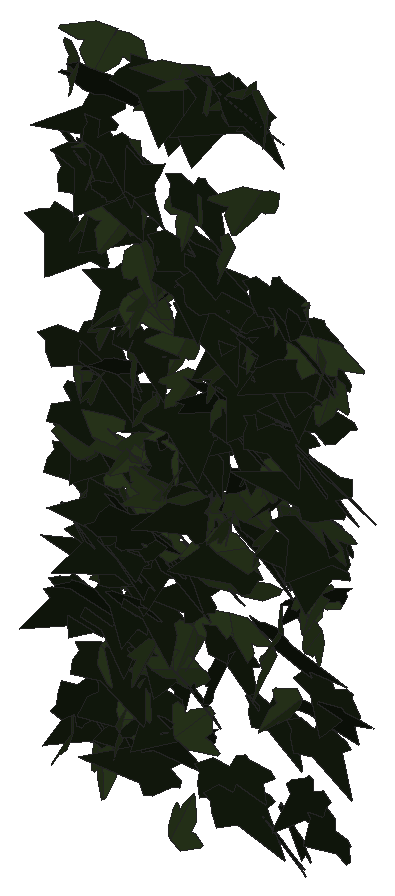
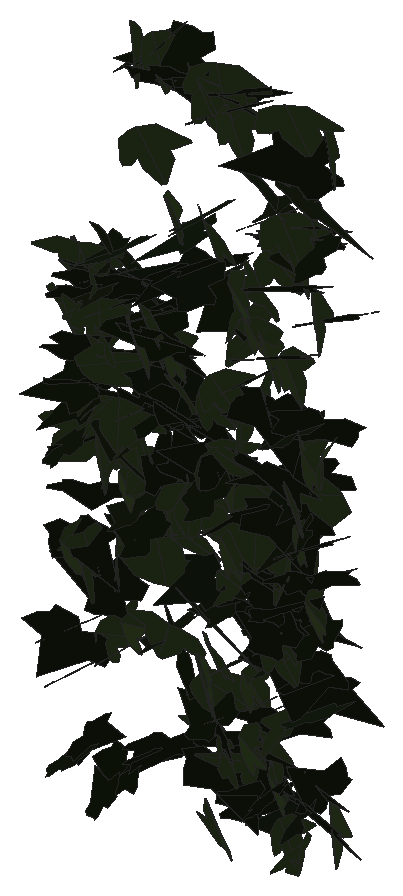
# SketchUp Ruby script. Lengths in millimetres.
U = 1.mm
M = Sketchup.active_model
def pt(a) = Geom::Point3d.new(a.map { |v| v * U })
def face(e, loops, mat)
  f = e.add_face(loops[0].map { |a| pt(a) })
  loops[1..].each { |l| e.add_face(l.map { |a| pt(a) }).erase! }
  f.material = f.back_material = mat if mat
  f
end
# faces: each face lists its corners as indices into pts; further lists are holes
def faces(e, pts, list, mat = nil) = list.each { |f| face(e, (f[0].is_a?(Array) ? f : [f]).map { |l| l.map { |i| pts[i] } }, mat) }
# xy, xz, yz: faces in a plane at the given z, y or x. An outline is a flat list of corners, or four numbers for a rectangle; further outlines are holes
def ring(l) = l.size == 4 ? [[l[0], l[1]], [l[2], l[1]], [l[2], l[3]], [l[0], l[3]]] : l.each_slice(2).to_a
def flat(e, list, mat, &to3) = list.each { |f| face(e, (f[0].is_a?(Array) ? f : [f]).map { |l| ring(l).map { |u, v| to3.(u, v) } }, mat) }
def xy(e, z, list, mat = nil) = flat(e, list, mat) { |x, y| [x, y, z] }
def xz(e, y, list, mat = nil) = flat(e, list, mat) { |x, z| [x, y, z] }
def yz(e, x, list, mat = nil) = flat(e, list, mat) { |y, z| [x, y, z] }
def lines(e, pts, list) = list.each { |a, b| e.add_line(pt(pts[a]), pt(pts[b])) }
# prism: a flat outline (further loops are holes) pulled along v
def prism(e, loops, v, mat = nil)
  f = face(e, loops, mat); d = Geom::Vector3d.new(v.map { |x| x * U })
  f.pushpull(f.normal.samedirection?(d) ? d.length : -d.length)
end
def box(e, o, s, mat = nil) = prism(e, [[o, [o[0] + s[0], o[1], o[2]], [o[0] + s[0], o[1] + s[1], o[2]], [o[0], o[1] + s[1], o[2]]]], [0, 0, s[2]], mat)
def at(x, y, z, deg = 0) = Geom::Transformation.translation(pt([x, y, z])) * Geom::Transformation.rotation(ORIGIN, Z_AXIS, deg.degrees)
def axes(o, x, y, z) = Geom::Transformation.new([*x, 0, *y, 0, *z, 0, *pt(o).to_a, 1])
def part(name) = M.definitions.add(name)
# library, detail: a bought-in or finely detailed component or shape, given as its bounding box
def library(name, o, s) = part(name).tap { |d| box(d.entities, o, s) }
def detail(e, o, s) = box(e.add_group.entities, o, s)
def put(e, d, t, mat = nil) = e.add_instance(d, t).tap { |i| i.material = mat if mat }
def group(e, t, mat = nil) = e.add_group.tap { |g| g.transformation = t; g.material = mat if mat }.entities
root = M.entities
M.materials.add("efeu1").color = [18, 25, 13]
M.materials.add("efeu2").color = [43, 57, 29]
c1 = part("ivyleaf_9")
p = [[39.1,54.8,31.7],[34.5,51.8,30.2],[-5.3,25.2,17.3],[-17.9,28.3,20.9],[-21.6,21.7,17],[-20.2,4.3,5.3],
  [-22.9,-0.3,2.5],[-17.1,-4,-0.6],[-2,-2.1,-1.2],[-0.7,-15.4,-10.1],[16.6,-22.3,-16.7],[21.1,-15.1,-12.5],
  [32.7,-10.7,-11],[46.1,-1.8,-6.6],[30.8,11.2,3.8]]
faces(c1.entities,p,[[0,1,2,3,4,5,6,7,8,9,10,11,12,13,14]],"efeu1")
c2 = part("ivyleaf_10")
p = [[0,12.8,-0.8],[-1.5,51.3,-10.9],[-4.9,51,-11.6],[-13.6,26.5,-7.3],[-13.2,15.9,-4.6],[-21.1,19.3,-7.2],
  [-29.5,16.3,-8.3],[-29.2,8.3,-6.2],[-19.7,-9.8,0.5],[-7.6,-13,4],[1,-12.2,5.8],[-0.4,51.1,-11.1],
  [-1.5,51.1,-10.9],[1,-12.4,5.9],[16.9,-12.4,3.5],[35.1,9.1,-5.1],[35,12.9,-6.1],[20.5,16.4,-4.9],
  [15.8,15,-3.8],[15.3,27.6,-7.1],[12.8,31.3,-7.8]]
faces(c2.entities,p,[[0,1,2,3,4,5,6,7,8,9,10],[11,12,0,13,14,15,16,17,18,19,20]],"efeu2")
put(root,c1,axes([3167.3,851.9,1947.2],[-1.71163,0.02943,0.11968],[-0.22866,-0.01275,-0.89967],[-0.05232,-0.90718,0.01653]))
put(root,c1,axes([3252.4,861.6,2324.2],[-0.11575,-0.94583,0.25251],[0.04501,-0.25434,-0.947],[1.8626,-0.05263,0.03857]))
put(root,c1,axes([3092.4,865,2330.9],[-0.99766,-0.72669,0.37742],[-0.1338,-0.40653,-0.8804],[1.55269,-0.50196,0.16664]))
put(root,c1,axes([3190,827.4,2438.5],[0.54104,0.53541,0.79457],[-0.52659,0.83937,-0.4666],[-1.74581,-0.08725,0.38698]))
put(root,c2,axes([3112.9,842.3,2090.9],[-0.7712,-0.10733,-1.03525],[1.96959,0.07673,-0.41303],[0.21089,-1.10908,0.07161]))
put(root,c2,axes([3164.4,858.5,2380.3],[-0.74877,-0.74862,0.505],[-0.03893,-0.54332,-0.82136],[1.71819,-0.33855,0.20146]))
put(root,c2,axes([3201.5,857.9,1829.8],[0.10736,-0.83868,0.42223],[0.20075,-0.41465,-0.83772],[1.77573,0.09758,0.06918]))
put(root,c2,axes([3199.2,856.4,2286.4],[0.21582,-0.91043,0.32112],[0.15942,-0.31283,-0.91651],[1.83043,0.13459,0.04196]))
put(root,c1,axes([3111.1,858.5,1856.1],[0.09211,0.1256,-0.88774],[-0.40662,-0.86181,-0.13358],[-1.65722,0.21844,-0.01657]))
put(root,c2,axes([3291,861.4,2056.1],[-0.08821,0.50692,-0.77285],[0.03891,-0.77307,-0.50829],[-1.75863,-0.04253,0.02752]))
put(root,c2,axes([3185.1,860,2333.8],[1.05203,-0.35932,0.77542],[1.2124,-0.44238,-0.65911],[1.08429,0.84328,-0.01536]))
put(root,c2,axes([3151.5,852.3,2249.2],[0.05261,-0.96666,0.06985],[0.05652,-0.069,-0.96666],[1.84368,0.0297,0.02764]))
put(root,c1,axes([3334.6,847.4,1688.7],[0.31329,-0.78141,-0.53609],[-0.03358,0.54149,-0.7947],[1.8032,0.14585,0.07834]))
put(root,c2,axes([3399.3,866.1,1822.8],[0.03799,-0.34084,0.87208],[0.19157,-0.86645,-0.34094],[1.77168,0.10099,0.01817]))
put(root,c2,axes([3134.6,847.1,2163.2],[0.242,-0.92573,-0.21991],[0.03708,0.22436,-0.93316],[1.8105,0.11914,0.04851]))
put(root,c2,axes([3218.8,843,2165.7],[-0.07443,-0.88003,-0.43626],[0.27149,0.42688,-0.87391],[1.84955,-0.09807,0.11072]))
put(root,c1,axes([3157.1,866.8,1871.5],[-0.13634,-0.73855,0.50918],[-0.10426,-0.50624,-0.742],[1.70409,-0.09006,-0.00466]))
put(root,c1,axes([3220.3,863.7,2574.1],[-0.82164,-0.93763,-0.01567],[0.09231,-0.0051,-1.03121],[1.78235,-0.43197,0.04618]))
put(root,c1,axes([3428.2,860.3,2277.4],[-1.7636,-0.19236,0.12728],[-0.23141,-0.04043,-0.94629],[0.37305,-0.93448,0.01474]))
put(root,c2,axes([3095.1,842,1687.4],[0.18402,-0.83212,-0.61124],[-0.10409,0.60893,-0.83762],[1.96229,0.11034,0.01289]))
put(root,c2,axes([3255,853.6,1741.5],[1.35818,-0.41325,-0.37001],[0.61897,-0.1767,0.82459],[-0.85519,-0.78419,0.00919]))
put(root,c1,axes([3169.3,841.5,1972.8],[-0.11479,-0.10418,0.94422],[1.73049,0.26763,0.08761],[-0.52352,0.9075,0.08256]))
put(root,c1,axes([3329,854.4,2597.8],[0.81855,-0.90853,-0.30046],[-0.25701,0.26849,-1.00517],[1.803,0.45074,-0.00687]))
put(root,c2,axes([3127.3,848.9,2445.7],[0.64331,-0.86532,-0.34696],[-0.13269,0.34457,-0.92727],[1.76936,0.34046,0.05661]))
put(root,c1,axes([3282.2,846.1,2369],[1.27105,-0.57956,-0.4415],[-0.26412,0.48676,-0.8489],[1.36123,0.63561,0.24754]))
put(root,c2,axes([3317.3,852.1,2387.8],[0.71463,-0.93857,-0.20251],[-0.08346,0.20046,-1.01035],[1.82548,0.37659,0.03309]))
put(root,c2,axes([3245.7,853.8,1608.1],[1.2389,-0.73981,-0.07337],[0.09338,-0.05456,0.98543],[-1.41184,-0.6528,0.00079]))
put(root,c1,axes([3320.2,870.3,1977.6],[-1.25451,-0.26857,0.61132],[-0.67706,-0.58569,-0.64089],[1.07542,-0.68203,0.30963]))
put(root,c1,axes([3277.3,854.5,2034],[-1.61102,0.36065,0.05804],[-0.10432,0.01943,-0.9201],[-0.68735,-0.84825,0.0036]))
put(root,c1,axes([3409.3,841.6,2308.2],[-0.85147,0.86442,0.32225],[-0.27728,0.28745,-0.97333],[-1.73373,-0.47051,-0.0026]))
put(root,c1,axes([3375.9,859,1813.1],[0.33026,-0.85237,-0.15761],[-0.0701,0.15334,-0.86984],[1.64824,0.17731,-0.00541]))
put(root,c2,axes([3351.6,860.1,2467.9],[-0.87179,-0.87367,0.30003],[-0.10421,-0.30863,-0.98229],[1.755,-0.45232,0.09071]))
put(root,c1,axes([3141.7,869.5,1973.7],[-0.77384,-0.07875,0.80711],[-1.07948,-0.61768,-0.346],[1.10307,-0.65971,0.22761]))
put(root,c2,axes([3182.1,853.8,2264.3],[0.35123,-0.94079,-0.16334],[-0.06352,0.15991,-0.95872],[1.81619,0.18753,-0.00194]))
put(root,c1,axes([3137.6,870.6,2431],[-1.24934,-0.74587,0.19918],[-0.11965,-0.20893,-0.98959],[1.4644,-0.6534,0.08907]))
put(root,c1,axes([3249.9,864.9,2150.7],[-0.42151,-0.95738,-0.12023],[0.06952,0.11495,-0.98262],[1.83508,-0.22426,0.00961]))
put(root,c1,axes([3154.8,858,1801.2],[-0.7348,-0.70133,-0.54457],[0.50248,0.47629,-0.80058],[1.61348,-0.46772,0.00131]))
put(root,c1,axes([3460.5,861.8,2113.7],[-1.09379,0.20172,0.72488],[-1.43095,-0.18893,-0.54353],[0.0549,-0.90556,0.27487]))
put(root,c1,axes([3284.4,860.7,2290.5],[-0.0781,-0.92797,-0.29273],[0.06005,0.29157,-0.92871],[1.85093,-0.04861,0.01778]))
put(root,c2,axes([3172.8,865.9,2209.4],[0.49749,-0.74865,0.54358],[0.6965,-0.43512,-0.77526],[1.6172,0.4177,0.16667]))
put(root,c1,axes([3129.1,869.2,2174],[0.10706,-0.89286,0.33367],[0.2883,-0.32163,-0.88618],[1.79102,0.10514,0.1227]))
put(root,c2,axes([3157.9,867.7,1721.2],[0.58031,-0.8303,0.57842],[0.53546,-0.51073,-0.88144],[1.84994,0.40829,0.07369]))
put(root,c1,axes([3442.1,870.7,2053.8],[-0.94354,-0.73784,0.29071],[-0.34205,-0.22939,-0.8887],[1.47006,-0.52695,-0.02019]))
put(root,c1,axes([3213.8,870.6,1672.6],[-0.65633,-0.2154,0.89744],[-1.49806,-0.4316,-0.40605],[0.91716,-0.8591,-0.02102]))
put(root,c1,axes([3138.3,870.2,2465.9],[0.07696,-0.98083,0.27735],[0.0741,-0.27588,-0.98131],[1.9385,0.04948,0.0265]))
put(root,c2,axes([3398.2,841.9,1927.7],[0.04753,-0.64407,-0.77364],[-0.04509,0.77329,-0.64454],[1.91533,0.03419,0.00403]))
put(root,c1,axes([3175.5,853.6,1927.4],[-0.95201,0.24562,0.72164],[-1.24926,0.3001,-0.55713],[-0.73769,-0.82518,0.01218]))
put(root,c1,axes([3266.8,867.8,2562.3],[-1.39976,-0.58268,-0.39107],[0.87444,0.02837,-0.90635],[1.00951,-0.8325,0.24283]))
put(root,c2,axes([3453.4,851.4,2287.6],[0.7031,-0.81428,-0.38138],[-0.09481,0.39315,-0.88766],[1.70867,0.35689,0.10768]))
put(root,c1,axes([3155.4,874.1,1923.6],[-0.14211,-0.66203,0.67681],[0.38742,-0.67426,-0.63708],[1.75973,0.09498,0.19492]))
put(root,c1,axes([3123.9,864.3,2423.5],[-0.3629,-0.88096,-0.41769],[0.84901,0.29961,-0.83555],[1.64992,-0.34794,0.33808]))
put(root,c1,axes([3236.5,868.8,1751.2],[-1.34148,-0.4847,0.14512],[-0.23564,-0.07607,-0.8554],[0.93367,-0.71561,-0.00737]))
put(root,c1,axes([3277,859.1,2598.4],[1.48359,-0.63543,0.21329],[0.42429,-0.06272,-1.00164],[1.20303,0.80574,0.09024]))
put(root,c2,axes([3188.9,865.4,2087.6],[0.54091,0.66329,-0.61443],[-0.85639,-0.45488,-0.69919],[-1.49254,0.50139,0.1785]))
put(root,c1,axes([3105.5,842.7,2122.5],[0.76819,-0.08687,-0.96647],[0.2857,1.03974,-0.03077],[1.82458,-0.12623,0.41173]))
put(root,c1,axes([3319.1,857.2,1713.6],[-0.07915,-0.76272,-0.61098],[-0.0113,0.61172,-0.76324],[1.8599,-0.02874,-0.03064]))
put(root,c1,axes([3184.1,869.4,2229.1],[0.03446,-0.95532,0.01024],[-0.01501,-0.01039,-0.95546],[1.81822,0.01802,-0.00808]))
put(root,c2,axes([3371.2,851.1,2590.5],[0.85035,-0.8008,-0.51243],[-0.02912,0.56007,-0.88859],[1.80917,0.38541,0.22655]))
put(root,c1,axes([3181.2,858.6,1725.8],[0.15181,-0.0846,-0.88803],[1.50845,0.41585,0.03158],[0.77907,-0.78869,0.1119]))
put(root,c1,axes([3135.8,850.1,1881],[1.42479,0.51234,-0.44094],[-0.71841,-0.22895,-0.9069],[-1.06721,0.83812,0.02181]))
put(root,c1,axes([3174.7,860.4,1740.8],[-1.52997,0.26072,0.29631],[-0.53692,0.09063,-0.84511],[-0.52532,-0.85196,0.00077]))
put(root,c1,axes([3282.8,864.3,1807],[0.09332,0.69244,0.79719],[-0.26305,-0.78697,0.69207],[1.99235,-0.13634,0.05403]))
put(root,c2,axes([3235.6,872.7,2115.5],[-0.85751,-0.48996,0.68573],[-0.30864,-0.71264,-0.61574],[1.57402,-0.40666,0.25285]))
put(root,c1,axes([3384.7,852.7,1658.8],[1.37861,-0.2885,-0.50061],[-0.87945,0.19267,-0.77967],[0.66014,0.85918,0.00675]))
put(root,c2,axes([3331.4,860.4,2596.1],[-0.31499,-0.98816,-0.04855],[0.02165,0.04732,-1.00192],[1.88281,-0.16586,0.0034]))
put(root,c1,axes([3227.6,876.2,2552.5],[-0.60418,-0.93045,0.24084],[-0.00022,-0.2536,-0.9799],[1.82919,-0.30736,0.07943]))
put(root,c2,axes([3237.1,859.1,2070],[0.40047,-0.88213,-0.16879],[-0.06727,0.16509,-0.90687],[1.70801,0.21333,0.00386]))
put(root,c1,axes([3176.4,871.8,2057.3],[1.09856,-0.78853,0.10991],[-0.11336,0.09261,0.9772],[-1.511,-0.58024,0.0066]))
put(root,c2,axes([3357.8,877.2,1855.2],[0.3772,-0.45252,0.84638],[0.62861,-0.77929,-0.49399],[1.71505,0.38516,-0.00509]))
put(root,c2,axes([3177.5,860.3,1763.6],[1.33941,-0.55614,-0.18043],[-0.14257,0.19425,-0.89095],[1.10358,0.70008,0.10388]))
put(root,c1,axes([3147.1,866.4,2448.6],[0.34081,-0.9602,-0.24181],[0.16139,0.2597,-0.96845],[1.87759,0.15197,0.12713]))
put(root,c2,axes([3317.7,866.5,1995.3],[-1.08032,0.02035,0.73262],[-1.25418,-0.41973,-0.49892],[0.61047,-0.8263,0.27148]))
put(root,c2,axes([3439,862.9,2300],[1.68427,0.37488,-0.01986],[-0.03513,-0.00735,-0.9611],[-0.71362,0.88516,0.00043]))
put(root,c2,axes([3082.7,880,2153.8],[-0.18559,-0.30544,0.97975],[1.05741,-0.84317,-0.20756],[1.64218,0.50841,0.24437]))
put(root,c2,axes([3092.9,854,2558.2],[0.67842,-0.77203,-0.55109],[-0.13965,0.56451,-0.83829],[1.79985,0.3348,0.14268]))
put(root,c1,axes([3101.4,847.5,1716.2],[-0.32365,-0.19771,0.96973],[1.30166,0.68771,0.26015],[-1.36142,0.70452,0.0182]))
put(root,c1,axes([3169.6,854.7,2192.9],[0.51905,0.88988,-0.32008],[-0.21093,-0.30076,-0.93058],[-1.78744,0.2939,0.01687]))
put(root,c2,axes([3246,868.4,1857.8],[1.08346,-0.68685,0.16456],[0.1919,-0.13016,-0.89209],[1.33045,0.57812,-0.00534]))
put(root,c1,axes([3392.9,876.4,2243.1],[-0.24293,-0.95999,0.10839],[-0.02176,-0.10782,-0.96843],[1.83853,-0.12812,0.00286]))
put(root,c1,axes([3098.1,860.3,2199.4],[-0.20051,-0.57039,-0.78902],[0.61026,0.72902,-0.56983],[1.74957,-0.31965,0.10833]))
put(root,c1,axes([3328.6,879.1,2145.1],[-0.27342,-0.92937,0.24009],[-0.04131,-0.23956,-0.94029],[1.82638,-0.14455,0.01468]))
put(root,c2,axes([3208.5,874.3,2330.9],[0.67473,-0.82101,0.41816],[0.30685,-0.38585,-0.89427],[1.72648,0.38944,-0.00448]))
put(root,c2,axes([3245.2,869.8,1814.5],[-0.77815,-0.20733,0.77898],[-1.26687,-0.40581,-0.45738],[0.8653,-0.78058,0.03088]))
put(root,c2,axes([3133.3,868.3,2404.1],[0.48862,-0.95513,0.03323],[0.01834,-0.03182,-0.98904],[1.81882,0.25691,0.00104]))
put(root,c2,axes([3312,861.5,2034.2],[0.06089,-0.9257,-0.29655],[0.05928,0.29753,-0.92542],[1.84904,0.02094,0.03944]))
put(root,c2,axes([3244.5,879,2101.5],[-0.33253,-0.69723,0.62679],[0.42333,-0.65021,-0.66127],[1.7334,0.02504,0.28174]))
put(root,c1,axes([3350.3,878.1,2206],[-1.26793,-0.65807,0.06911],[-0.08278,-0.05431,-0.93639],[1.25659,-0.66758,0.00805]))
put(root,c1,axes([3300.7,875.7,1864.2],[0.39157,-0.92635,0.10949],[0.03475,-0.1081,-0.94891],[1.77497,0.20648,-0.00558]))
put(root,c2,axes([3243,878,2184.1],[-0.18578,-0.81256,0.56907],[0.12047,-0.57576,-0.81124],[1.88415,-0.0433,0.10798]))
put(root,c2,axes([3301.2,872.7,2227.2],[0.12605,-0.95926,0.25328],[0.04318,-0.25231,-0.96153],[1.88773,0.06983,0.00508]))
put(root,c1,axes([3117.1,869.5,1705.4],[-1.58696,0.27462,-0.12822],[0.22319,-0.05375,-0.87778],[-0.53188,-0.84193,0.01421]))
put(root,c1,axes([3321.6,878,2571.8],[-1.79176,-0.31371,0.20184],[-0.3392,-0.10309,-0.9915],[0.62368,-0.9573,0.04062]))
put(root,c2,axes([3189.7,852.7,2277],[0.60501,0.67844,0.62044],[0.17932,0.62899,-0.73606],[-1.74052,0.30063,0.13983]))
put(root,c2,axes([3428.1,863.9,2072.4],[-1.81813,0.2278,-0.36849],[0.68157,-0.0868,-0.98209],[-0.46395,-1.02022,0.00128]))
put(root,c2,axes([3364.7,873.7,2033.3],[0.31468,-0.90004,0.23776],[0.08891,-0.23316,-0.9151],[1.76949,0.17178,0.0037]))
put(root,c1,axes([3390.8,875.5,2309.7],[0.82557,-0.86158,0.16841],[0.1273,-0.15486,-0.96457],[1.66594,0.4388,-0.00975]))
put(root,c2,axes([3238.3,867.7,2591.6],[-1.3798,-0.71478,0.07784],[-0.09951,-0.05784,-1.01809],[1.36479,-0.72686,0.00447]))
put(root,c2,axes([3265.3,872.4,2575],[1.1516,-0.80814,0.14738],[0.24215,-0.08864,-1.00841],[1.54455,0.61643,0.04821]))
put(root,c2,axes([3211.5,878.8,2021.5],[-1.17495,-0.50673,-0.6516],[-0.91738,-0.43923,0.79826],[-1.27531,0.78281,0.0261]))
put(root,c1,axes([3166.2,885.9,2266.2],[-1.2758,-0.58293,0.40505],[-0.22083,-0.45964,-0.85352],[1.33279,-0.63416,0.24631]))
put(root,c1,axes([3375.9,872.3,2171.7],[-0.07485,-0.90661,-0.33703],[0.01673,0.33696,-0.90745],[1.84076,-0.03993,-0.00546]))
put(root,c1,axes([3369.9,877.8,1886.6],[0.65147,-0.47171,0.80009],[1.00282,-0.60357,-0.58128],[1.45568,0.62691,0.04237]))
put(root,c1,axes([3261.4,858.6,2072.6],[-1.26816,-0.14142,0.80916],[1.49837,0.18726,0.68106],[-0.44595,1.03134,-0.01271]))
put(root,c2,axes([3302.6,869.5,2176.8],[1.18713,-0.71751,-0.12292],[-0.08502,0.12384,-0.94956],[1.38285,0.62357,0.04714]))
put(root,c2,axes([3332.5,863.2,2068.4],[-1.12401,-0.61552,-0.4088],[0.62428,0.25054,-0.85112],[1.26012,-0.67316,0.05702]))
put(root,c1,axes([3085.3,884.5,1930.4],[1.19497,-0.5745,-0.46011],[0.73872,-0.25542,0.84858],[-1.19022,-0.73532,0.06473]))
put(root,c1,axes([3253.2,879.8,2123.3],[0.12814,-0.97691,0.01161],[0.00173,-0.01157,-0.97922],[1.85938,0.06734,0.00011]))
put(root,c2,axes([3099.2,881.7,2156],[0.21797,-0.81074,0.55762],[0.47337,-0.5193,-0.80612],[1.81193,0.2332,0.14352]))
put(root,c2,axes([3240.9,874.9,2566.2],[-0.69476,-0.92195,0.21443],[0.00894,-0.23158,-0.98771],[1.80146,-0.35441,0.0876]))
put(root,c2,axes([3179.7,857.3,1730.7],[0.33003,-0.14546,-0.96569],[1.62105,0.50234,0.07728],[0.90925,-0.84279,0.21274]))
put(root,c1,axes([3198.5,870.2,1975.5],[-1.55506,0.37026,0.15557],[-0.27836,0.05411,-0.89699],[-0.71186,-0.82999,0.01092]))
put(root,c1,axes([3326.7,871.6,2138.7],[1.36267,-0.66448,0.00847],[0.01207,-0.00562,-0.97682],[1.26469,0.71602,0.0002]))
put(root,c1,axes([3167,890.2,1695.8],[-0.51198,-0.33244,0.91473],[-0.85745,-0.79869,-0.42277],[1.64191,-0.52076,0.06445]))
put(root,c1,axes([3147.2,888,2363.1],[-1.3238,-0.5992,0.35237],[-0.19183,-0.40628,-0.88983],[1.30899,-0.66552,0.22596]))
put(root,c1,axes([3188.9,883,1874],[-0.05213,-0.93466,0.14007],[0.03814,-0.14068,-0.93475],[1.7983,-0.02411,0.02389]))
put(root,c2,axes([3149.2,877,1902.3],[-0.38364,-0.8945,0.24019],[-0.06123,-0.2389,-0.9167],[1.76165,-0.2031,0.02044]))
put(root,c2,axes([3215.2,873.2,2548.7],[-0.30034,-1.0057,0.01739],[-0.03497,-0.01472,-1.01789],[1.91402,-0.15808,-0.01587]))
put(root,c1,axes([3411.1,888.6,1700.4],[0.0504,-0.14233,-0.90205],[0.75228,-0.81173,0.13968],[-1.56678,-0.39432,0.03805]))
put(root,c1,axes([3131.9,885.4,1835.7],[-0.16991,-0.92092,0.19135],[-0.01518,-0.19146,-0.92518],[1.79006,-0.08904,0.01032]))
put(root,c2,axes([3144.8,857.8,1801.2],[0.05694,0.83877,0.57828],[-0.04884,0.57896,-0.83844],[-1.93835,0.01005,0.03811]))
put(root,c2,axes([3278.8,872.2,2046.1],[-1.16204,-0.69177,-0.01816],[0.02452,0.01285,-0.92268],[1.31681,-0.6107,0.00115]))
put(root,c1,axes([3234.9,868.6,1722],[0.13416,0.8965,-0.45168],[-0.15036,-0.44643,-0.89842],[-1.90461,0.09839,0.03911]))
put(root,c1,axes([3307.2,884.7,2058.2],[0.42586,0.39828,0.90514],[-0.82069,-0.79584,0.45679],[1.69369,-0.48577,-0.00625]))
put(root,c1,axes([3169.8,878.7,1937],[-1.29115,-0.40843,-0.53311],[0.83322,0.30566,-0.7913],[0.96923,-0.80686,-0.02992]))
put(root,c1,axes([3410.7,882.6,2016.8],[-0.94414,-0.72428,-0.23086],[0.33217,0.15979,-0.87635],[1.40813,-0.52332,0.05193]))
put(root,c1,axes([3091.4,893.5,1835],[-0.7459,-0.63578,0.60141],[-0.07228,-0.64598,-0.70765],[1.66403,-0.31305,0.23884]))
put(root,c1,axes([3284.9,877.2,2177.2],[-0.15923,0.64711,-0.67817],[-0.04549,-0.68212,-0.64793],[-1.78343,-0.04038,0.07708]))
put(root,c1,axes([3235,876.2,2361.7],[0.162,-0.87813,-0.43831],[0.13877,0.44439,-0.87616],[1.86271,0.04326,0.1034]))
put(root,c1,axes([3280.4,869.9,2330.9],[0.26495,-0.73438,-0.69502],[-0.02894,0.69998,-0.74267],[1.92416,0.11165,0.08453]))
put(root,c1,axes([3115.4,880.3,1693.7],[0.99139,-0.72414,0.12094],[0.11372,-0.10598,-0.89194],[1.39264,0.52415,-0.01326]))
put(root,c2,axes([3183,886.9,1770],[0.33448,-0.74951,0.53474],[0.29515,-0.51252,-0.76934],[1.72727,0.23272,0.02791]))
put(root,c2,axes([3309.4,877.9,1940.6],[-1.79344,-0.44249,0.09803],[0.17415,0.03576,1.04103],[-0.84481,0.94674,0.0065]))
put(root,c1,axes([3135.4,886.6,1961.9],[0.39145,-0.38388,0.87576],[0.96549,-0.71552,-0.43278],[1.54261,0.54524,0.04864]))
put(root,c1,axes([3102.4,893.5,2047],[-0.80983,-0.70439,0.44819],[-0.2178,-0.44909,-0.81444],[1.57396,-0.42456,0.1179]))
put(root,c2,axes([3217.3,856.5,2291.9],[-0.06369,0.04377,0.99083],[-0.7847,0.90105,-0.05373],[-1.71675,-0.41348,-0.0122]))
put(root,c1,axes([3411.4,887.3,2267.9],[-1.11398,-0.77968,-0.08939],[0.08093,0.07984,-0.97484],[1.49142,-0.5867,-0.01387]))
put(root,c1,axes([3389.9,876.1,2096.9],[-0.96063,0.75424,-0.39077],[0.42741,-0.31989,-0.90751],[-1.55917,-0.55239,-0.00802]))
put(root,c2,axes([3117.4,879.9,1654.8],[0.17462,0.92056,-0.34703],[-0.11091,-0.34284,-0.92485],[-1.86907,0.10635,0.02246]))
put(root,c1,axes([3225.2,891.4,1783.4],[0.34242,-0.66315,0.67163],[0.45376,-0.62962,-0.68554],[1.73808,0.29502,0.04666]))
put(root,c1,axes([3278.6,880.3,2173.5],[0.74909,-0.47353,0.75117],[1.37416,-0.3076,-0.57223],[0.98371,0.79029,0.22736]))
put(root,c1,axes([3124.9,875.1,2487.8],[-1.3433,0.71174,-0.00258],[-0.2647,-0.14148,-0.98254],[-1.32848,-0.69149,0.19838]))
put(root,c1,axes([3227.1,854.8,2301],[0.49546,0.54478,0.78932],[0.55268,0.73472,-0.60287],[-1.73963,0.38858,0.03327]))
put(root,c2,axes([3110.4,880.8,2055.5],[0.15065,-0.92586,0.10516],[0.04668,-0.10343,-0.92911],[1.77281,0.0814,0.01553]))
put(root,c1,axes([3416,879.3,2143.8],[1.3771,-0.65778,0.07693],[0.12181,-0.04395,-0.97781],[1.25451,0.72632,0.0105]))
put(root,c2,axes([3125.2,884.2,2587.4],[-1.57819,-0.45287,0.31982],[-0.18759,-0.44583,-0.88686],[1.03835,-0.76886,0.32588]))
put(root,c2,axes([3391.1,861.6,2250.8],[-0.12082,-0.33137,-0.92792],[1.06782,0.75222,-0.30701],[1.54154,-0.54703,0.13994]))
put(root,c2,axes([3131.4,888.2,1925.5],[0.84701,-0.46695,0.62702],[0.9147,-0.40564,-0.64322],[1.17353,0.6532,0.0488]))
put(root,c1,axes([3437,897.2,1657.3],[-0.61495,-0.36797,0.79211],[-0.30166,-0.80585,-0.43901],[1.63467,-0.28714,0.21697]))
put(root,c1,axes([3092.6,872.2,2531.6],[1.72668,-0.10553,0.4551],[0.86062,-0.05131,-0.91337],[0.22331,1.0137,0.00114]))
put(root,c1,axes([3204.1,886.1,1938.7],[0.74713,-0.82947,0.10242],[0.07327,-0.09509,-0.91765],[1.58894,0.39441,-0.00584]))
put(root,c2,axes([3267.5,876.9,2035.3],[-1.60702,0.29558,-0.21811],[0.3682,-0.10696,-0.8939],[-0.59432,-0.86551,0.03597]))
put(root,c2,axes([3381.6,878.7,2123.8],[-0.6327,-0.84368,-0.23717],[0.90946,0.03813,-0.80546],[1.39817,-0.40659,0.4166]))
put(root,c1,axes([3194.6,895.7,1808.3],[-0.51218,-0.78092,0.38916],[-0.05113,-0.39964,-0.82053],[1.65978,-0.25329,0.09481]))
put(root,c1,axes([3078.4,886.9,2425.4],[0.96474,-0.83393,0.20261],[0.20027,-0.17314,-0.9759],[1.62098,0.51771,-0.00002]))
put(root,c2,axes([3093.8,874.9,2352.4],[0.28848,-0.92217,-0.3501],[0.04856,0.35776,-0.93129],[1.87668,0.1325,0.07792]))
put(root,c1,axes([3140.2,872.9,2072.3],[0.57539,0.76918,-0.4325],[-0.52777,-0.35121,-0.81844],[-1.59437,0.39385,0.11484]))
put(root,c2,axes([3233.5,888.2,2407.9],[1.33201,-0.70381,0.33659],[0.43807,-0.24578,-0.99251],[1.41869,0.7367,-0.00956]))
put(root,c2,axes([3174.5,880.9,2035.2],[1.66616,0.50343,0.02185],[0.03377,0.01297,-1.00988],[-0.95843,0.87563,0.0024]))
put(root,c1,axes([3433.4,899,2058.2],[-0.17014,-0.58409,0.72232],[-0.02082,-0.72494,-0.58756],[1.76781,-0.06476,0.0626]))
put(root,c2,axes([3084.6,892.5,1976.8],[0.51451,-0.74396,0.51626],[0.37159,-0.47821,-0.79138],[1.68288,0.33304,0.0169]))
put(root,c2,axes([3129.3,886,2446.3],[-0.91466,-0.84701,0.21226],[-0.05656,-0.22628,-0.97024],[1.66091,-0.47415,0.08385]))
put(root,c2,axes([3213.6,889.8,1743.5],[0.9399,-0.61224,0.49872],[0.82194,-0.28304,-0.77513],[1.25819,0.64226,0.13381]))
put(root,c1,axes([3357.1,885.9,2338],[0.56104,-0.9262,-0.20577],[0.1081,0.23231,-0.96431],[1.80249,0.27435,0.12188]))
put(root,c2,axes([3427.3,875.6,1919.4],[0.94191,-0.6377,-0.44423],[-0.24873,0.45086,-0.79283],[1.45805,0.48887,0.15172]))
put(root,c1,axes([3418.2,887.8,1783.2],[0.32973,-0.91476,-0.16218],[0.00273,0.16524,-0.93048],[1.76812,0.17034,0.03168]))
put(root,c1,axes([3270,875.6,1913.7],[-1.22036,0.69311,0.21821],[-0.28317,0.15962,-0.94422],[-1.35365,-0.65825,0.0008]))
put(root,c2,axes([3439.5,886.2,2241.8],[1.47268,-0.54789,0.07739],[0.12565,-0.04067,-0.94811],[1.04557,0.77659,0.00494]))
put(root,c1,axes([3225.7,895.1,2068.9],[0.6583,-0.79676,0.44921],[0.28707,-0.424,-0.86817],[1.71696,0.37638,-0.02708]))
put(root,c2,axes([3127.2,889.3,1681.1],[-0.26464,-0.85619,0.22979],[0.17149,-0.24505,-0.8585],[1.67843,-0.10996,0.12395]))
put(root,c1,axes([3232.2,865.4,2098.6],[0.19609,0.10914,0.98023],[1.41038,0.6418,-0.14935],[-1.23868,0.74804,-0.01488]))
put(root,c2,axes([3344.7,880.3,2098.1],[-1.17753,0.66022,0.22592],[-0.72612,-0.06725,-0.84832],[-1.11197,-0.65522,0.31471]))
put(root,c1,axes([3142.5,881.7,1938.8],[-1.45563,-0.53418,0.18892],[0.32055,0.08868,0.93262],[-1.02962,0.78281,0.02326]))
put(root,c1,axes([3327.4,891.8,2158.4],[-1.79559,-0.08712,-0.10658],[0.2103,-0.0391,-0.94621],[0.15622,-0.94865,0.04879]))
put(root,c1,axes([3328.8,896.2,2018.9],[0.41866,-0.89706,0.27124],[0.14036,-0.26118,-0.9236],[1.77809,0.23184,0.00904]))
put(root,c2,axes([3217.9,895.8,2219],[-0.5451,-0.80362,0.4711],[0.18836,-0.51633,-0.8206],[1.76285,-0.19332,0.23335]))
put(root,c1,axes([3163.7,878.3,2070.8],[0.56926,-0.58484,-0.6619],[0.03725,0.70304,-0.61235],[1.68061,0.18252,0.23777]))
put(root,c1,axes([3410.2,882.9,2132.4],[1.35207,-0.60476,-0.29924],[-0.44674,0.18587,-0.93292],[1.20396,0.74813,-0.01012]))
put(root,c1,axes([3237.8,893.3,2425.4],[0.34217,-0.96531,-0.07932],[0.00478,0.08114,-0.98176],[1.84337,0.17897,0.01727]))
put(root,c2,axes([3369.1,884.3,2129],[-1.67265,-0.3293,0.02358],[-0.04188,-0.00846,-0.93853],[0.62693,-0.87914,0.0002]))
put(root,c1,axes([3312.7,900,1991.3],[0.59145,-0.74062,0.5461],[0.3869,-0.5069,-0.80314],[1.70803,0.37128,-0.00717]))
put(root,c1,axes([3107.3,882.4,2064.2],[1.19579,-0.58568,-0.45673],[-0.62218,0.31909,-0.8589],[1.26924,0.7082,0.00927]))
put(root,c2,axes([3371.2,880.2,2074.2],[-0.53783,0.92203,0.14813],[-0.07986,0.14207,-0.96436],[-1.77551,-0.28569,-0.0015]))
put(root,c1,axes([3086.8,894.4,2020],[-0.58314,-0.87543,-0.31963],[0.25477,0.29163,-0.92707],[1.7553,-0.33316,0.02837]))
put(root,c2,axes([3290.7,889.6,1877.9],[1.74055,-0.01963,0.28681],[0.54559,-0.00966,-0.91474],[0.04115,0.95841,-0.00335]))
put(root,c2,axes([3124.9,886.9,2113.2],[0.71283,-0.85823,-0.17643],[-0.1055,0.16828,-0.93626],[1.6642,0.37828,0.01622]))
put(root,c1,axes([3239.1,892.3,2337.4],[1.28498,-0.64526,0.39472],[0.63782,-0.21915,-0.93149],[1.2906,0.75075,0.06735]))
put(root,c1,axes([3218.9,896.4,1789],[-0.80732,0.20028,-0.78486],[1.38608,-0.29349,-0.46851],[-0.67478,-0.84249,-0.02336]))
put(root,c1,axes([3374.6,904.6,1633.4],[0.05899,-0.43481,0.73962],[0.02701,-0.73974,-0.43548],[1.63266,0.02795,-0.01952]))
put(root,c2,axes([3389.3,894.1,2221.4],[1.12314,-0.67433,0.32163],[0.62952,-0.13169,-0.88299],[1.27494,0.65906,0.15265]))
put(root,c1,axes([3292.2,906.6,2287.1],[-0.70112,-0.80212,0.38113],[-0.00161,-0.41231,-0.86855],[1.69017,-0.33313,0.15728]))
put(root,c1,axes([3234.1,887.4,1962.2],[1.47338,-0.49636,-0.12358],[-0.23249,0.03829,-0.91901],[0.94535,0.78303,-0.0334]))
put(root,c1,axes([3429.9,905.4,1834.5],[-0.45762,-0.75901,0.39154],[-0.11044,-0.39131,-0.79419],[1.62168,-0.24084,0.0564]))
put(root,c2,axes([3391.6,886.1,2073.8],[0.26427,-0.89862,-0.26963],[0.05221,0.27634,-0.90685],[1.78482,0.12497,0.06645]))
put(root,c2,axes([3342,888.9,2242.1],[0.449,-0.93089,-0.15971],[-0.10835,0.1503,-0.96015],[1.79429,0.24202,-0.01802]))
put(root,c1,axes([3427.7,880,1822.5],[1.57121,0.26468,-0.13252],[-0.23701,-0.04563,-0.86693],[-0.51107,0.83488,-0.00537]))
put(root,c1,axes([3126.6,900.7,1925.5],[0.40878,-0.3171,0.87041],[0.85583,-0.74548,-0.38255],[1.54141,0.498,-0.01843]))
put(root,c1,axes([3382.9,897.3,2297.7],[-1.07426,-0.70278,-0.37824],[0.53879,0.25685,-0.8997],[1.42018,-0.62905,0.05521]))
put(root,c2,axes([3385.5,901.7,2186.2],[0.27947,0.32298,0.89101],[-0.81895,-0.78063,0.35388],[1.60711,-0.45396,0.02539]))
put(root,c2,axes([3249.4,884.2,1843.5],[0.46158,-0.82501,-0.4338],[-0.22811,0.41692,-0.85992],[1.75926,0.27052,0.00232]))
put(root,c2,axes([3391.1,888.5,2249.2],[-0.98974,-0.8198,-0.09776],[0.08694,0.08678,-0.9708],[1.56888,-0.52198,-0.00787]))
put(root,c1,axes([3430.7,902.2,2198.6],[-1.32558,-0.26249,0.58932],[-1.06026,-0.19263,-0.74421],[0.61917,-0.8918,-0.01271]))
put(root,c1,axes([3288.5,891.3,2257.7],[1.4034,-0.47364,0.36848],[0.66253,-0.13789,-0.87387],[0.93028,0.81272,0.06648]))
put(root,c1,axes([3150.4,897.5,2138.5],[-1.69989,-0.12559,-0.3101],[0.58366,0.0461,-0.90196],[0.25457,-0.94435,-0.00279]))
put(root,c2,axes([3394.5,872,2287.2],[0.2199,0.59728,-0.82362],[0.25394,0.81285,0.6082],[1.91958,-0.17596,0.01389]))
put(root,c2,axes([3135.7,881.7,2015.8],[-0.99694,0.71468,0.32697],[-0.41028,0.24721,-0.88571],[-1.43841,-0.56585,0.02602]))
put(root,c1,axes([3317.9,899.3,2249.4],[-1.77089,-0.15791,0.00198],[-0.0018,-0.00629,-0.94377],[0.30055,-0.93046,0.00604]))
put(root,c1,axes([3421.7,891,1961],[-0.10393,0.72871,-0.52813],[0.00696,-0.52891,-0.73018],[-1.7128,-0.04637,0.02908]))
put(root,c1,axes([3370.5,895.6,2289.9],[0.75589,-0.89256,-0.12893],[-0.01005,0.13858,-0.9756],[1.71632,0.39391,0.05107]))
put(root,c2,axes([3203.4,874.9,1957.9],[0.59742,0.61788,-0.69707],[0.41779,0.6658,0.68901],[1.72289,-0.3757,0.07463]))
put(root,c2,axes([3325.9,885.4,2261],[0.76219,-0.74693,-0.47849],[-0.34557,0.44485,-0.84639],[1.65248,0.43754,0.0437]))
put(root,c2,axes([3200.5,899.3,2019.5],[0.1958,-0.85252,0.32302],[0.25169,-0.30768,-0.85414],[1.71672,0.14234,0.08838]))
put(root,c2,axes([3418.6,906.8,1948.9],[0.2868,-0.54383,0.75517],[0.34812,-0.73277,-0.5642],[1.73659,0.23671,-0.01162]))
put(root,c2,axes([3409.8,893.5,1956.7],[0.45981,0.82501,-0.27116],[-0.34945,-0.22657,-0.85293],[-1.61543,0.28384,0.10732]))
